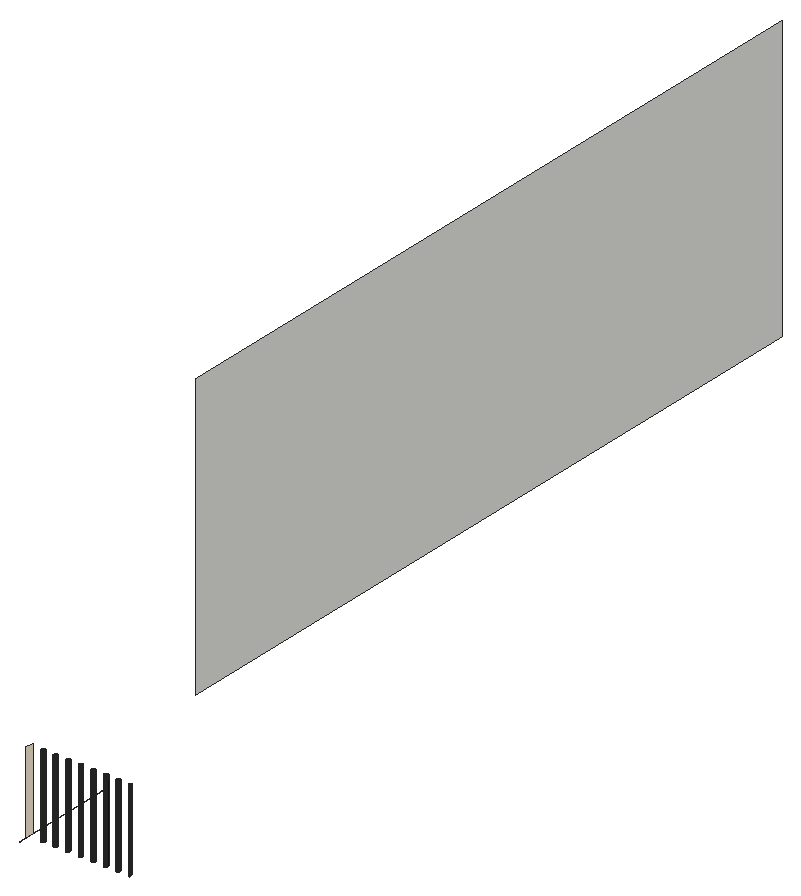
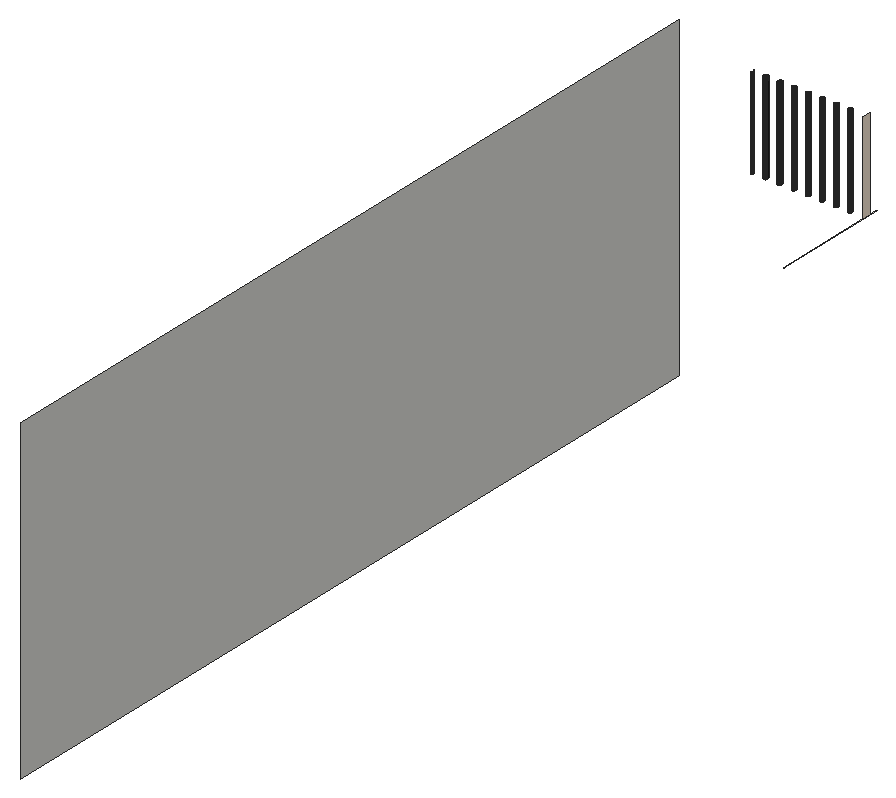
# SketchUp Ruby script. Lengths in inches.
U = 1.inch
M = Sketchup.active_model
def pt(a) = Geom::Point3d.new(a.map { |v| v * U })
def face(e, loops, mat)
  f = e.add_face(loops[0].map { |a| pt(a) })
  loops[1..].each { |l| e.add_face(l.map { |a| pt(a) }).erase! }
  f.material = f.back_material = mat if mat
  f
end
# faces: each face lists its corners as indices into pts; further lists are holes
def faces(e, pts, list, mat = nil) = list.each { |f| face(e, (f[0].is_a?(Array) ? f : [f]).map { |l| l.map { |i| pts[i] } }, mat) }
# xy, xz, yz: faces in a plane at the given z, y or x. An outline is a flat list of corners, or four numbers for a rectangle; further outlines are holes
def ring(l) = l.size == 4 ? [[l[0], l[1]], [l[2], l[1]], [l[2], l[3]], [l[0], l[3]]] : l.each_slice(2).to_a
def flat(e, list, mat, &to3) = list.each { |f| face(e, (f[0].is_a?(Array) ? f : [f]).map { |l| ring(l).map { |u, v| to3.(u, v) } }, mat) }
def xy(e, z, list, mat = nil) = flat(e, list, mat) { |x, y| [x, y, z] }
def xz(e, y, list, mat = nil) = flat(e, list, mat) { |x, z| [x, y, z] }
def yz(e, x, list, mat = nil) = flat(e, list, mat) { |y, z| [x, y, z] }
def lines(e, pts, list) = list.each { |a, b| e.add_line(pt(pts[a]), pt(pts[b])) }
# prism: a flat outline (further loops are holes) pulled along v
def prism(e, loops, v, mat = nil)
  f = face(e, loops, mat); d = Geom::Vector3d.new(v.map { |x| x * U })
  f.pushpull(f.normal.samedirection?(d) ? d.length : -d.length)
end
def box(e, o, s, mat = nil) = prism(e, [[o, [o[0] + s[0], o[1], o[2]], [o[0] + s[0], o[1] + s[1], o[2]], [o[0], o[1] + s[1], o[2]]]], [0, 0, s[2]], mat)
def at(x, y, z, deg = 0) = Geom::Transformation.translation(pt([x, y, z])) * Geom::Transformation.rotation(ORIGIN, Z_AXIS, deg.degrees)
def axes(o, x, y, z) = Geom::Transformation.new([*x, 0, *y, 0, *z, 0, *pt(o).to_a, 1])
def part(name) = M.definitions.add(name)
# library, detail: a bought-in or finely detailed component or shape, given as its bounding box
def library(name, o, s) = part(name).tap { |d| box(d.entities, o, s) }
def detail(e, o, s) = box(e.add_group.entities, o, s)
def put(e, d, t, mat = nil) = e.add_instance(d, t).tap { |i| i.material = mat if mat }
def group(e, t, mat = nil) = e.add_group.tap { |g| g.transformation = t; g.material = mat if mat }.entities
root = M.entities
M.materials.add("[0028_AntiqueWhite]").color = [250, 235, 215]
M.materials.add("[Color M08]").color = [30, 30, 30]
xy(root,321,[[50.7,190.5,50.75,190.5,50.75,231.9375]])
xy(root,321,[[55.99,194.51,55.8,194.57,55.63,194.67,55.5,194.81,55.41,194.99,55.36,195.18,55.37,195.375,55.42,195.5625,55.53,195.73,55.67,195.86,55.84,195.95,56.03,196,56.23,195.99,56.42,195.9375,56.58,195.83,56.72,195.69,56.81,195.52,56.85,195.33,56.85,195.13,56.79,194.95,56.6875,194.78,56.55,194.64,56.375,194.55,56.18,194.51],[61.05,194.51,60.86,194.57,60.7,194.67,60.5625,194.81,60.47,194.99,60.42,195.18,60.43,195.375,60.49,195.5625,60.59,195.73,60.73,195.86,60.9,195.95,61.1,196,61.29,195.99,61.48,195.9375,61.65,195.83,61.78,195.69,61.87,195.52,61.92,195.33,61.91,195.13,61.85,194.95,61.75,194.78,61.61,194.64,61.4375,194.55,61.25,194.51],[66.11,194.51,65.93,194.57,65.76,194.67,65.625,194.81,65.53,194.99,65.49,195.18,65.49,195.375,65.55,195.5625,65.65,195.73,65.79,195.86,65.97,195.95,66.16,196,66.35,195.99,66.54,195.9375,66.71,195.83,66.84,195.69,66.93,195.52,66.98,195.33,66.97,195.13,66.92,194.95,66.8125,194.78,66.67,194.64,66.5,194.55,66.31,194.51],[71.18,194.51,70.99,194.57,70.82,194.67,70.6875,194.81,70.59,194.99,70.55,195.18,70.56,195.375,70.61,195.5625,70.71,195.73,70.86,195.86,71.03,195.95,71.22,196,71.42,195.99,71.6,195.9375,71.77,195.83,71.9,195.69,72,195.52,72.04,195.33,72.04,195.13,71.98,194.95,71.875,194.78,71.73,194.64,71.5625,194.55,71.37,194.51],[76.24,194.51,76.05,194.57,75.88,194.67,75.75,194.81,75.66,194.99,75.61,195.18,75.62,195.375,75.67,195.5625,75.78,195.73,75.92,195.86,76.09,195.95,76.28,196,76.48,195.99,76.67,195.9375,76.83,195.83,76.97,195.69,77.06,195.52,77.1,195.33,77.1,195.13,77.04,194.95,76.9375,194.78,76.8,194.64,76.625,194.55,76.43,194.51],
  [81.3,194.51,81.11,194.57,80.95,194.67,80.8125,194.81,80.72,194.99,80.67,195.18,80.68,195.375,80.74,195.5625,80.84,195.73,80.98,195.86,81.15,195.95,81.35,196,81.54,195.99,81.73,195.9375,81.9,195.83,82.03,195.69,82.12,195.52,82.17,195.33,82.16,195.13,82.1,194.95,82,194.78,81.86,194.64,81.6875,194.55,81.5,194.51],[86.36,194.51,86.18,194.57,86.01,194.67,85.875,194.81,85.78,194.99,85.74,195.18,85.74,195.375,85.8,195.5625,85.9,195.73,86.04,195.86,86.22,195.95,86.41,196,86.6,195.99,86.79,195.9375,86.96,195.83,87.09,195.69,87.18,195.52,87.23,195.33,87.22,195.13,87.17,194.95,87.0625,194.78,86.92,194.64,86.75,194.55,86.56,194.51]],"[Color M08]")
xz(root,194.51,[[55.99,321,56.18,353.72],[61.05,321,61.25,353.72],[66.11,321,66.31,353.72],[71.18,321,71.37,353.72],[76.24,321,76.43,353.72],
  [81.3,321,81.5,353.72],[86.36,321,86.56,353.72]],"[Color M08]")
yz(root,35.1875,[[298.4375,321,592.9375,435]])
yz(root,50.75,[[193.51,321,196.625,353.72]],"[0028_AntiqueWhite]")
yz(root,56.85,[[195.13,321,195.33,353.72]],"[Color M08]")
yz(root,65.49,[[195.18,321,195.375,353.72]],"[Color M08]")
yz(root,72.04,[[195.13,321,195.33,353.72]],"[Color M08]")
yz(root,77.1,[[195.13,321,195.33,353.72]],"[Color M08]")
yz(root,85.74,[[195.18,321,195.375,353.72]],"[Color M08]")
p = [[55.8,194.57,321],[55.99,194.51,321],[55.99,194.51,353.72],[55.8,194.57,353.72],[56.18,194.51,321],[56.375,194.55,321],
  [56.375,194.55,353.72],[56.18,194.51,353.72],[60.86,194.57,321],[61.05,194.51,321],[61.05,194.51,353.72],[60.86,194.57,353.72],
  [61.25,194.51,321],[61.4375,194.55,321],[61.4375,194.55,353.72],[61.25,194.51,353.72],[65.93,194.57,321],[66.11,194.51,321],
  [66.11,194.51,353.72],[65.93,194.57,353.72],[66.31,194.51,321],[66.5,194.55,321],[66.5,194.55,353.72],[66.31,194.51,353.72],
  [70.99,194.57,321],[71.18,194.51,321],[71.18,194.51,353.72],[70.99,194.57,353.72],[71.37,194.51,321],[71.5625,194.55,321],
  [71.5625,194.55,353.72],[71.37,194.51,353.72],[76.05,194.57,321],[76.24,194.51,321],[76.24,194.51,353.72],[76.05,194.57,353.72],
  [76.43,194.51,321],[76.625,194.55,321],[76.625,194.55,353.72],[76.43,194.51,353.72],[81.11,194.57,321],[81.3,194.51,321],
  [81.3,194.51,353.72],[81.11,194.57,353.72],[81.5,194.51,321],[81.6875,194.55,321],[81.6875,194.55,353.72],[81.5,194.51,353.72],
  [86.18,194.57,321],[86.36,194.51,321],[86.36,194.51,353.72],[86.18,194.57,353.72],[86.56,194.51,321],[86.75,194.55,321],
  [86.75,194.55,353.72],[86.56,194.51,353.72],[91.24,194.57,321],[91.43,194.51,321],[91.43,194.51,353.72],[91.24,194.57,353.72],
  [55.63,194.67,321],[55.63,194.67,353.72],[56.55,194.64,321],[56.55,194.64,353.72],[56.6875,194.78,321],[56.6875,194.78,353.72],
  [60.7,194.67,321],[60.7,194.67,353.72],[61.61,194.64,321],[61.61,194.64,353.72],[61.75,194.78,321],[61.75,194.78,353.72],
  [65.76,194.67,321],[65.76,194.67,353.72],[66.67,194.64,321],[66.67,194.64,353.72],[66.8125,194.78,321],[66.8125,194.78,353.72],
  [70.82,194.67,321],[70.82,194.67,353.72],[71.73,194.64,321],[71.73,194.64,353.72],[71.875,194.78,321],[71.875,194.78,353.72],
  [75.88,194.67,321],[75.88,194.67,353.72],[76.8,194.64,321],[76.8,194.64,353.72],[76.9375,194.78,321],[76.9375,194.78,353.72],
  [80.95,194.67,321],[80.95,194.67,353.72],[81.86,194.64,321],[81.86,194.64,353.72],[82,194.78,321],[82,194.78,353.72],
  [86.01,194.67,321],[86.01,194.67,353.72],[86.92,194.64,321],[86.92,194.64,353.72],[87.0625,194.78,321],[87.0625,194.78,353.72],
  [91.07,194.67,321],[91.07,194.67,353.72],[55.5,194.81,321],[55.5,194.81,353.72],[60.5625,194.81,321],[60.5625,194.81,353.72],
  [65.625,194.81,321],[65.625,194.81,353.72],[70.6875,194.81,321],[70.6875,194.81,353.72],[75.75,194.81,321],[75.75,194.81,353.72],
  [80.8125,194.81,321],[80.8125,194.81,353.72],[85.875,194.81,321],[85.875,194.81,353.72],[90.9375,194.81,321],[90.9375,194.81,353.72],
  [55.41,194.99,321],[55.41,194.99,353.72],[56.79,194.95,321],[56.79,194.95,353.72],[60.47,194.99,321],[60.47,194.99,353.72],
  [61.85,194.95,321],[61.85,194.95,353.72],[65.53,194.99,321],[65.53,194.99,353.72],[66.92,194.95,321],[66.92,194.95,353.72],
  [70.59,194.99,321],[70.59,194.99,353.72],[71.98,194.95,321],[71.98,194.95,353.72],[75.66,194.99,321],[75.66,194.99,353.72],
  [77.04,194.95,321],[77.04,194.95,353.72],[80.72,194.99,321],[80.72,194.99,353.72],[82.1,194.95,321],[82.1,194.95,353.72],
  [85.78,194.99,321],[85.78,194.99,353.72],[87.17,194.95,321],[87.17,194.95,353.72],[90.84,194.99,321],[90.84,194.99,353.72],
  [56.85,195.13,321],[56.85,195.13,353.72],[61.91,195.13,321],[61.91,195.13,353.72],[66.97,195.13,321],[66.97,195.13,353.72],
  [72.04,195.13,321],[72.04,195.13,353.72],[77.1,195.13,321],[77.1,195.13,353.72],[82.16,195.13,321],[82.16,195.13,353.72],
  [87.22,195.13,321],[87.22,195.13,353.72],[55.36,195.18,321],[55.36,195.18,353.72],[60.42,195.18,321],[60.42,195.18,353.72],
  [65.49,195.18,321],[65.49,195.18,353.72],[70.55,195.18,321],[70.55,195.18,353.72],[75.61,195.18,321],[75.61,195.18,353.72],
  [80.67,195.18,321],[80.67,195.18,353.72],[85.74,195.18,321],[85.74,195.18,353.72],[90.8,195.18,321],[90.8,195.18,353.72],
  [61.92,195.33,321],[61.92,195.33,353.72],[66.98,195.33,321],[66.98,195.33,353.72],[82.17,195.33,321],[82.17,195.33,353.72],
  [87.23,195.33,321],[87.23,195.33,353.72],[55.37,195.375,321],[55.37,195.375,353.72],[60.43,195.375,321],[60.43,195.375,353.72],
  [70.56,195.375,321],[70.56,195.375,353.72],[75.62,195.375,321],[75.62,195.375,353.72],[80.68,195.375,321],[80.68,195.375,353.72],
  [90.81,195.375,321],[90.81,195.375,353.72],[56.85,195.33,321],[56.81,195.52,321],[56.81,195.52,353.72],[56.85,195.33,353.72],
  [61.87,195.52,321],[61.87,195.52,353.72],[66.93,195.52,321],[66.93,195.52,353.72],[72.04,195.33,321],[72,195.52,321],
  [72,195.52,353.72],[72.04,195.33,353.72],[77.1,195.33,321],[77.06,195.52,321],[77.06,195.52,353.72],[77.1,195.33,353.72],
  [82.12,195.52,321],[82.12,195.52,353.72],[87.18,195.52,321],[87.18,195.52,353.72],[55.42,195.5625,321],[55.42,195.5625,353.72],
  [60.49,195.5625,321],[60.49,195.5625,353.72],[65.55,195.5625,321],[65.49,195.375,321],[65.49,195.375,353.72],[65.55,195.5625,353.72],
  [70.61,195.5625,321],[70.61,195.5625,353.72],[75.67,195.5625,321],[75.67,195.5625,353.72],[80.74,195.5625,321],[80.74,195.5625,353.72],
  [85.8,195.5625,321],[85.74,195.375,321],[85.74,195.375,353.72],[85.8,195.5625,353.72],[90.86,195.5625,321],[90.86,195.5625,353.72],
  [56.72,195.69,321],[56.72,195.69,353.72],[61.78,195.69,321],[61.78,195.69,353.72],[66.84,195.69,321],[66.84,195.69,353.72],
  [71.9,195.69,321],[71.9,195.69,353.72],[76.97,195.69,321],[76.97,195.69,353.72],[82.03,195.69,321],[82.03,195.69,353.72],
  [87.09,195.69,321],[87.09,195.69,353.72],[55.53,195.73,321],[55.53,195.73,353.72],[60.59,195.73,321],[60.59,195.73,353.72],
  [65.65,195.73,321],[65.65,195.73,353.72],[70.71,195.73,321],[70.71,195.73,353.72],[75.78,195.73,321],[75.78,195.73,353.72],
  [80.84,195.73,321],[80.84,195.73,353.72],[85.9,195.73,321],[85.9,195.73,353.72],[90.96,195.73,321],[90.96,195.73,353.72],
  [55.67,195.86,321],[55.67,195.86,353.72],[56.58,195.83,321],[56.58,195.83,353.72],[60.73,195.86,321],[60.73,195.86,353.72],
  [61.65,195.83,321],[61.65,195.83,353.72],[65.79,195.86,321],[65.79,195.86,353.72],[66.71,195.83,321],[66.71,195.83,353.72],
  [70.86,195.86,321],[70.86,195.86,353.72],[71.77,195.83,321],[71.77,195.83,353.72],[75.92,195.86,321],[75.92,195.86,353.72],
  [76.83,195.83,321],[76.83,195.83,353.72],[80.98,195.86,321],[80.98,195.86,353.72],[81.9,195.83,321],[81.9,195.83,353.72],
  [86.04,195.86,321],[86.04,195.86,353.72],[86.96,195.83,321],[86.96,195.83,353.72],[91.11,195.86,321],[91.11,195.86,353.72],
  [56.42,195.9375,321],[56.42,195.9375,353.72],[61.48,195.9375,321],[61.48,195.9375,353.72],[66.54,195.9375,321],[66.54,195.9375,353.72],
  [71.6,195.9375,321],[71.6,195.9375,353.72],[76.67,195.9375,321],[76.67,195.9375,353.72],[81.73,195.9375,321],[81.73,195.9375,353.72],
  [86.79,195.9375,321],[86.79,195.9375,353.72],[55.84,195.95,321],[55.84,195.95,353.72],[56.23,195.99,321],[56.23,195.99,353.72],
  [60.9,195.95,321],[60.9,195.95,353.72],[61.29,195.99,321],[61.29,195.99,353.72],[65.97,195.95,321],[65.97,195.95,353.72],
  [66.35,195.99,321],[66.35,195.99,353.72],[71.03,195.95,321],[71.03,195.95,353.72],[71.42,195.99,321],[71.42,195.99,353.72],
  [76.09,195.95,321],[76.09,195.95,353.72],[76.48,195.99,321],[76.48,195.99,353.72],[81.15,195.95,321],[81.15,195.95,353.72],
  [81.54,195.99,321],[81.54,195.99,353.72],[86.22,195.95,321],[86.22,195.95,353.72],[86.6,195.99,321],[86.6,195.99,353.72],
  [91.28,195.95,321],[91.28,195.95,353.72],[56.03,196,321],[56.03,196,353.72],[61.1,196,321],[61.1,196,353.72],
  [66.16,196,321],[66.16,196,353.72],[71.22,196,321],[71.22,196,353.72],[76.28,196,321],[76.28,196,353.72],
  [81.35,196,321],[81.35,196,353.72],[86.41,196,321],[86.41,196,353.72]]
faces(root,p,[[0,1,2,3],[4,5,6,7],[8,9,10,11],[12,13,14,15],[16,17,18,19],[20,21,22,23],[24,25,26,27],[28,29,30,31],
  [32,33,34,35],[36,37,38,39],[40,41,42,43],[44,45,46,47],[48,49,50,51],[52,53,54,55],[56,57,58,59],[60,0,3,61],
  [5,62,63,6],[62,64,65,63],[66,8,11,67],[13,68,69,14],[68,70,71,69],[72,16,19,73],[21,74,75,22],[74,76,77,75],
  [78,24,27,79],[29,80,81,30],[80,82,83,81],[84,32,35,85],[37,86,87,38],[86,88,89,87],[90,40,43,91],[45,92,93,46],
  [92,94,95,93],[96,48,51,97],[53,98,99,54],[98,100,101,99],[102,56,59,103],[104,60,61,105],[106,66,67,107],[108,72,73,109],
  [110,78,79,111],[112,84,85,113],[114,90,91,115],[116,96,97,117],[118,102,103,119],[120,104,105,121],[64,122,123,65],[124,106,107,125],
  [70,126,127,71],[128,108,109,129],[76,130,131,77],[132,110,111,133],[82,134,135,83],[136,112,113,137],[88,138,139,89],[140,114,115,141],
  [94,142,143,95],[144,116,117,145],[100,146,147,101],[148,118,119,149],[122,150,151,123],[126,152,153,127],[130,154,155,131],[134,156,157,135],
  [138,158,159,139],[142,160,161,143],[146,162,163,147],[164,120,121,165],[166,124,125,167],[168,128,129,169],[170,132,133,171],[172,136,137,173],
  [174,140,141,175],[176,144,145,177],[178,148,149,179],[152,180,181,153],[154,182,183,155],[160,184,185,161],[162,186,187,163],[188,164,165,189],
  [190,166,167,191],[192,170,171,193],[194,172,173,195],[196,174,175,197],[198,178,179,199],[200,201,202,203],[180,204,205,181],[182,206,207,183],
  [208,209,210,211],[212,213,214,215],[184,216,217,185],[186,218,219,187],[220,188,189,221],[222,190,191,223],[224,225,226,227],[228,192,193,229],
  [230,194,195,231],[232,196,197,233],[234,235,236,237],[238,198,199,239],[201,240,241,202],[204,242,243,205],[206,244,245,207],[209,246,247,210],
  [213,248,249,214],[216,250,251,217],[218,252,253,219],[254,220,221,255],[256,222,223,257],[258,224,227,259],[260,228,229,261],[262,230,231,263],
  [264,232,233,265],[266,234,237,267],[268,238,239,269],[270,254,255,271],[240,272,273,241],[274,256,257,275],[242,276,277,243],[278,258,259,279],
  [244,280,281,245],[282,260,261,283],[246,284,285,247],[286,262,263,287],[248,288,289,249],[290,264,265,291],[250,292,293,251],[294,266,267,295],
  [252,296,297,253],[298,268,269,299],[272,300,301,273],[276,302,303,277],[280,304,305,281],[284,306,307,285],[288,308,309,289],[292,310,311,293],
  [296,312,313,297],[314,270,271,315],[300,316,317,301],[318,274,275,319],[302,320,321,303],[322,278,279,323],[304,324,325,305],[326,282,283,327],
  [306,328,329,307],[330,286,287,331],[308,332,333,309],[334,290,291,335],[310,336,337,311],[338,294,295,339],[312,340,341,313],[342,298,299,343],
  [344,314,315,345],[316,344,345,317],[346,318,319,347],[320,346,347,321],[348,322,323,349],[324,348,349,325],[350,326,327,351],[328,350,351,329],
  [352,330,331,353],[332,352,353,333],[354,334,335,355],[336,354,355,337],[356,338,339,357],[340,356,357,341]],"[Color M08]")
